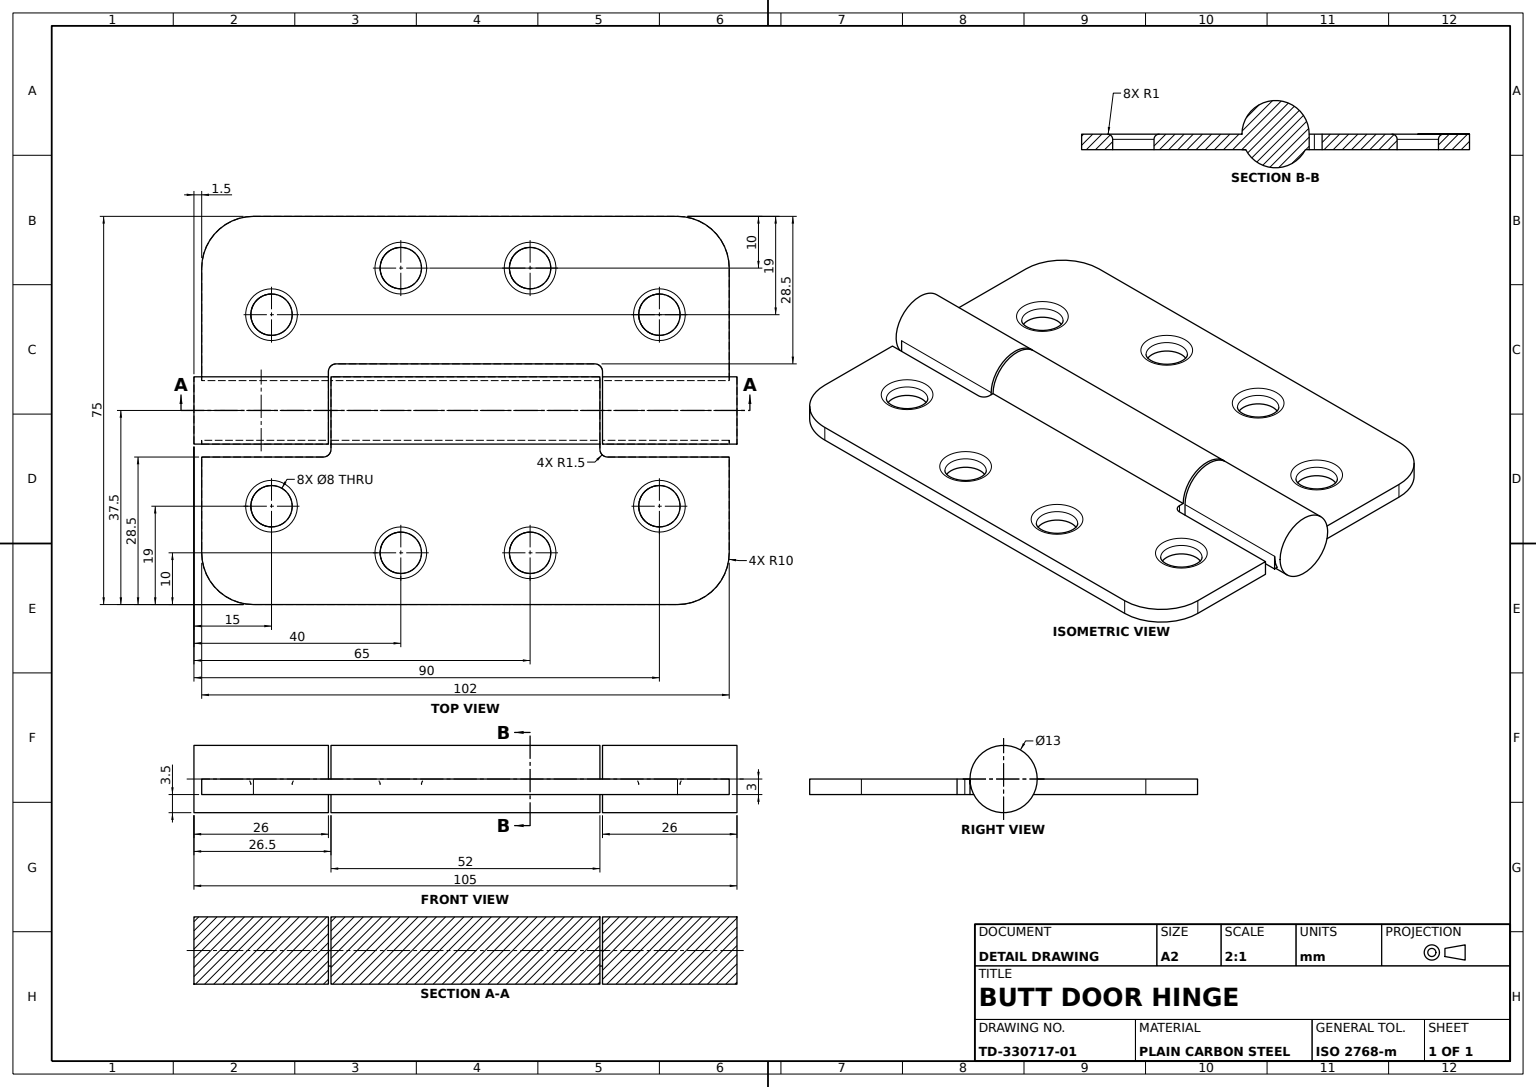
solid
v1 (77.5,-3,-5.766281)
v2 (77.5,-3,5.766281)
e1 v1 v2 CIRCLE(AX(P(77.5,0,0),D(-1,0,0),D(0,0,1)),6.5)
v3 (102,-3,-5.766281)
e2 v1 v3 LINE
v4 (102,0,-6.5)
e3 v4 v3 CIRCLE(AX(P(102,0,0),D(-1,0,0),D(0,0,-1)),6.5)
v5 (103.5,0,-6.5)
e4 v5 v4 LINE
v6 (103.5,0,6.5)
e5 v5 v6 CIRCLE(AX(P(103.5,0,0),D(-1,0,0),D(0,0,1)),6.5)
v7 (102,0,6.5)
e6 v6 v7 LINE
v8 (102,-3,5.766281)
e7 v8 v7 CIRCLE(AX(P(102,0,0),D(-1,0,0),D(0,0,-1)),6.5)
e8 v8 v2 LINE
face CYL(AX(P(77.5,0,0),D(-1,0,0),D(0,0,1)),6.5) [-e1 e2 -e3 -e4 e5 e6 -e7 e8]
v9 (77.5,-3,6.5)
v10 (102,-3,6.5)
e9 v9 v10 LINE
e10 v2 v9 LINE
e11 v10 v8 LINE
face PLANE(AX(P(26,-3,-7.5),D(0,1,0),D(0,0,1))) rev [-e9 -e10 -e8 -e11]
v11 (88.5,-1,-14.5)
v12 (88.5,-1,-22.5)
e12 v11 v12 CIRCLE(AX(P(88.5,-1,-18.5),D(0,1,0),D(0,0,1)),4)
v13 (88.5,-3,-22.5)
e13 v13 v12 LINE
v14 (88.5,-3,-14.5)
e14 v14 v13 CIRCLE(AX(P(88.5,-3,-18.5),D(0,1,0),D(0,0,1)),4)
e15 v14 v11 LINE
face CYL(AX(P(88.5,-3,-18.5),D(0,1,0),D(0,0,1)),4) rev [e12 -e13 -e14 e15]
v15 (13.5,-1,-14.5)
v16 (13.5,-1,-22.5)
e16 v15 v16 CIRCLE(AX(P(13.5,-1,-18.5),D(0,1,0),D(0,0,1)),4)
v17 (13.5,-3,-22.5)
e17 v17 v16 LINE
v18 (13.5,-3,-14.5)
e18 v18 v17 CIRCLE(AX(P(13.5,-3,-18.5),D(0,1,0),D(0,0,1)),4)
e19 v18 v15 LINE
face CYL(AX(P(13.5,-3,-18.5),D(0,1,0),D(0,0,1)),4) rev [e16 -e17 -e18 e19]
v19 (0,-3,5.766281)
v20 (24.5,-3,5.766281)
e20 v19 v20 LINE
v21 (0,0,6.5)
e21 v19 v21 CIRCLE(AX(P(0,0,0),D(-1,0,0),D(0,0,1)),6.5)
v22 (24.5,0,6.5)
e22 v21 v22 LINE
v23 (24.5,6.5,0)
e23 v23 v22 CIRCLE(AX(P(24.5,0,0),D(1,0,0),D(0,1,0)),6.5)
v24 (-1.5,6.5,0)
e24 v24 v23 LINE
v25 (-1.5,-6.5,0)
e25 v24 v25 CIRCLE(AX(P(-1.5,0,0),D(1,0,0),D(0,1,0)),6.5)
v26 (24.5,-6.5,0)
e26 v25 v26 LINE
e27 v20 v26 CIRCLE(AX(P(24.5,0,0),D(1,0,0),D(0,1,0)),6.5)
face CYL(AX(P(24.5,0,0),D(1,0,0),D(0,1,0)),6.5) [-e20 e21 e22 -e23 -e24 e25 e26 -e27]
v27 (26,-3,-9)
v28 (26,0,-9)
e28 v27 v28 LINE
v29 (24.5,0,-7.5)
e29 v29 v28 CIRCLE(AX(P(26,0,-7.5),D(0,-1,0),D(0,0,1)),1.5)
v30 (24.5,-3,-7.5)
e30 v30 v29 LINE
e31 v30 v27 CIRCLE(AX(P(26,-3,-7.5),D(0,-1,0),D(0,0,1)),1.5)
face CYL(AX(P(26,-3,-7.5),D(0,1,0),D(0,0,1)),1.5) rev [e28 -e29 -e30 e31]
v31 (63.5,-3,-31.5)
v32 (63.5,-1,-31.5)
e32 v31 v32 LINE
v33 (63.5,-3,-23.5)
e33 v33 v31 CIRCLE(AX(P(63.5,-3,-27.5),D(0,1,0),D(0,0,1)),4)
v34 (63.5,-1,-23.5)
e34 v33 v34 LINE
e35 v34 v32 CIRCLE(AX(P(63.5,-1,-27.5),D(0,1,0),D(0,0,1)),4)
face CYL(AX(P(63.5,-3,-27.5),D(0,1,0),D(0,0,1)),4) rev [-e32 -e33 e34 e35]
v35 (24.5,-3,-5.766281)
e36 v26 v35 CIRCLE(AX(P(24.5,0,0),D(1,0,0),D(0,1,0)),6.5)
e37 v35 v30 LINE
v36 (24.5,0,-6.5)
e38 v36 v29 LINE
e39 v36 v23 CIRCLE(AX(P(24.5,0,0),D(1,0,0),D(0,1,0)),6.5)
v37 (24.5,-3,6.5)
e40 v37 v22 LINE
e41 v37 v20 LINE
face PLANE(AX(P(24.5,-3,6.5),D(1,0,0),D(0,0,-1))) [e36 e37 e30 -e38 e39 e23 -e40 e41 e27]
v38 (0,-3,6.5)
e42 v38 v37 LINE
e43 v38 v21 LINE
face PLANE(AX(P(0,-3,6.5),D(0,0,1),D(1,0,0))) [e42 e40 -e22 -e43]
e44 v12 v11 CIRCLE(AX(P(88.5,-1,-18.5),D(0,1,0),D(0,0,1)),4)
v39 (88.5,0,-23.5)
e45 v39 v12 CIRCLE(AX(P(88.5,-1,-23.5),D(1,0,0),D(0,0,-1)),1)
v40 (88.5,0,-13.5)
e46 v40 v39 CIRCLE(AX(P(88.5,0,-18.5),D(0,-1,0),D(0,0,1)),5)
e47 v40 v11 CIRCLE(AX(P(88.5,-1,-13.5),D(-1,0,0),D(0,0,1)),1)
face TORUS(AX(P(88.5,-1,-18.5),D(0,1,0),D(0,0,1)),5,1) [-e44 -e45 -e46 e47]
v41 (38.5,-3,-23.5)
v42 (38.5,-3,-31.5)
e48 v41 v42 CIRCLE(AX(P(38.5,-3,-27.5),D(0,1,0),D(0,0,1)),4)
v43 (38.5,-1,-23.5)
e49 v41 v43 LINE
v44 (38.5,-1,-31.5)
e50 v43 v44 CIRCLE(AX(P(38.5,-1,-27.5),D(0,1,0),D(0,0,1)),4)
e51 v42 v44 LINE
face CYL(AX(P(38.5,-3,-27.5),D(0,1,0),D(0,0,1)),4) rev [-e48 e49 e50 -e51]
e52 v44 v43 CIRCLE(AX(P(38.5,-1,-27.5),D(0,1,0),D(0,0,1)),4)
e53 v42 v41 CIRCLE(AX(P(38.5,-3,-27.5),D(0,1,0),D(0,0,1)),4)
face CYL(AX(P(38.5,-3,-27.5),D(0,1,0),D(0,0,1)),4) rev [e51 e52 -e49 -e53]
v45 (0,0,-6.5)
e54 v36 v45 LINE
v46 (0,-3,-5.766281)
e55 v45 v46 CIRCLE(AX(P(0,0,0),D(-1,0,0),D(0,0,1)),6.5)
e56 v35 v46 LINE
e57 v25 v24 CIRCLE(AX(P(-1.5,0,0),D(1,0,0),D(0,1,0)),6.5)
face CYL(AX(P(24.5,0,0),D(1,0,0),D(0,1,0)),6.5) [-e39 e54 e55 -e56 -e36 -e26 e57 e24]
e58 v13 v14 CIRCLE(AX(P(88.5,-3,-18.5),D(0,1,0),D(0,0,1)),4)
face CYL(AX(P(88.5,-3,-18.5),D(0,1,0),D(0,0,1)),4) rev [-e15 -e58 e13 e44]
v47 (63.5,0,-22.5)
v48 (63.5,0,-32.5)
e59 v47 v48 CIRCLE(AX(P(63.5,0,-27.5),D(0,-1,0),D(0,0,1)),5)
e60 v47 v34 CIRCLE(AX(P(63.5,-1,-22.5),D(-1,0,0),D(0,0,1)),1)
e61 v32 v34 CIRCLE(AX(P(63.5,-1,-27.5),D(0,1,0),D(0,0,1)),4)
e62 v48 v32 CIRCLE(AX(P(63.5,-1,-32.5),D(1,0,0),D(0,0,-1)),1)
face TORUS(AX(P(63.5,-1,-27.5),D(0,1,0),D(0,0,1)),5,1) [-e59 e60 -e61 -e62]
v49 (76,0,-9)
e63 v28 v49 LINE
v50 (76,-3,-9)
e64 v27 v50 LINE
e65 v50 v49 LINE
face PLANE(AX(P(26,-3,-9),D(0,0,1),D(1,0,0))) [-e63 -e28 e64 e65]
v51 (10,-3,-37.5)
v52 (10,0,-37.5)
e66 v51 v52 LINE
v53 (92,0,-37.5)
e67 v53 v52 LINE
v54 (92,-3,-37.5)
e68 v54 v53 LINE
e69 v54 v51 LINE
face PLANE(AX(P(92,-3,-37.5),D(0,0,-1),D(-1,0,0))) [e66 -e67 -e68 e69]
v55 (0,0,-27.5)
e70 v55 v45 LINE
v56 (0,-3,-27.5)
e71 v56 v55 LINE
e72 v56 v46 LINE
face PLANE(AX(P(0,-3,0),D(-1,0,0),D(0,0,1))) [-e70 -e71 e72 -e55]
e73 v19 v38 LINE
face PLANE(AX(P(0,-3,0),D(-1,0,0),D(0,0,1))) [e73 e43 -e21]
face PLANE(AX(P(-1.5,0,0),D(-1,0,0),D(0,-1,0))) [-e57 -e25]
e74 v48 v47 CIRCLE(AX(P(63.5,0,-27.5),D(0,-1,0),D(0,0,1)),5)
face TORUS(AX(P(63.5,-1,-27.5),D(0,1,0),D(0,0,1)),5,1) [-e35 -e60 -e74 e62]
e75 v10 v7 LINE
v57 (77.5,0,6.5)
e76 v57 v7 LINE
e77 v9 v57 LINE
face PLANE(AX(P(77.5,-3,6.5),D(0,0,1),D(1,0,0))) [e75 -e76 -e77 e9]
e78 v52 v55 CIRCLE(AX(P(10,0,-27.5),D(0,1,0),D(0,0,1)),10)
e79 v51 v56 CIRCLE(AX(P(10,-3,-27.5),D(0,1,0),D(0,0,1)),10)
face CYL(AX(P(10,-3,-27.5),D(0,1,0),D(0,0,1)),10) [e71 -e78 -e66 e79]
face PLANE(AX(P(26,-3,-7.5),D(0,1,0),D(0,0,1))) rev [e20 -e41 -e42 -e73]
v58 (77.5,-3,-7.5)
e80 v50 v58 CIRCLE(AX(P(76,-3,-7.5),D(0,-1,0),D(0,0,1)),1.5)
v59 (77.5,0,-7.5)
e81 v58 v59 LINE
e82 v49 v59 CIRCLE(AX(P(76,0,-7.5),D(0,-1,0),D(0,0,1)),1.5)
face CYL(AX(P(76,-3,-7.5),D(0,1,0),D(0,0,1)),1.5) rev [e80 e81 -e82 -e65]
v60 (77.5,0,-6.5)
e83 v57 v60 CIRCLE(AX(P(77.5,0,0),D(-1,0,0),D(0,0,1)),6.5)
e84 v6 v5 CIRCLE(AX(P(103.5,0,0),D(-1,0,0),D(0,0,1)),6.5)
e85 v60 v4 LINE
face CYL(AX(P(77.5,0,0),D(-1,0,0),D(0,0,1)),6.5) [-e83 e76 -e6 e84 e4 -e85]
e86 v17 v18 CIRCLE(AX(P(13.5,-3,-18.5),D(0,1,0),D(0,0,1)),4)
e87 v16 v15 CIRCLE(AX(P(13.5,-1,-18.5),D(0,1,0),D(0,0,1)),4)
face CYL(AX(P(13.5,-3,-18.5),D(0,1,0),D(0,0,1)),4) rev [-e19 -e86 e17 e87]
e88 v39 v40 CIRCLE(AX(P(88.5,0,-18.5),D(0,-1,0),D(0,0,1)),5)
v61 (13.5,0,-13.5)
v62 (13.5,0,-23.5)
e89 v61 v62 CIRCLE(AX(P(13.5,0,-18.5),D(0,-1,0),D(0,0,1)),5)
e90 v62 v61 CIRCLE(AX(P(13.5,0,-18.5),D(0,-1,0),D(0,0,1)),5)
e91 v59 v60 LINE
v63 (102,0,-27.5)
e92 v4 v63 LINE
e93 v63 v53 CIRCLE(AX(P(92,0,-27.5),D(0,1,0),D(0,0,1)),10)
v64 (38.5,0,-22.5)
v65 (38.5,0,-32.5)
e94 v64 v65 CIRCLE(AX(P(38.5,0,-27.5),D(0,-1,0),D(0,0,1)),5)
e95 v65 v64 CIRCLE(AX(P(38.5,0,-27.5),D(0,-1,0),D(0,0,1)),5)
face PLANE(AX(P(26,0,-7.5),D(0,1,0),D(0,0,1))) [e88 e46] [e59 e74] [e89 e90] [e63 e82 e91 e85 e92 e93 e67 e78 e70 -e54 e38 e29] [e94 e95]
e96 v62 v16 CIRCLE(AX(P(13.5,-1,-23.5),D(1,0,0),D(0,0,-1)),1)
e97 v61 v15 CIRCLE(AX(P(13.5,-1,-13.5),D(-1,0,0),D(0,0,1)),1)
face TORUS(AX(P(13.5,-1,-18.5),D(0,1,0),D(0,0,1)),5,1) [-e87 -e96 -e89 e97]
e98 v58 v1 LINE
face PLANE(AX(P(77.5,-3,-7.5),D(-1,0,0),D(0,0,1))) [e10 e77 e83 -e91 -e81 e98 e1]
e99 v31 v33 CIRCLE(AX(P(63.5,-3,-27.5),D(0,1,0),D(0,0,1)),4)
face CYL(AX(P(63.5,-3,-27.5),D(0,1,0),D(0,0,1)),4) rev [-e99 e32 e61 -e34]
e100 v64 v43 CIRCLE(AX(P(38.5,-1,-22.5),D(-1,0,0),D(0,0,1)),1)
e101 v65 v44 CIRCLE(AX(P(38.5,-1,-32.5),D(1,0,0),D(0,0,-1)),1)
face TORUS(AX(P(38.5,-1,-27.5),D(0,1,0),D(0,0,1)),5,1) [-e50 -e100 -e95 e101]
face TORUS(AX(P(13.5,-1,-18.5),D(0,1,0),D(0,0,1)),5,1) [-e16 -e97 -e90 e96]
v66 (102,-3,-27.5)
e102 v66 v63 LINE
e103 v66 v54 CIRCLE(AX(P(92,-3,-27.5),D(0,1,0),D(0,0,1)),10)
face CYL(AX(P(92,-3,-27.5),D(0,1,0),D(0,0,1)),10) [-e93 -e102 e103 e68]
e104 v3 v66 LINE
face PLANE(AX(P(26,-3,-7.5),D(0,1,0),D(0,0,1))) rev [e18 e86] [e99 e33] [e58 e14] [-e72 -e79 -e69 -e103 -e104 -e2 -e98 -e80 -e64 -e31 -e37 e56] [e48 e53]
face PLANE(AX(P(102,-3,6.5),D(1,0,0),D(0,0,-1))) [e11 e7 -e75]
face PLANE(AX(P(103.5,0,0),D(-1,0,0),D(0,0,1))) rev [-e84 -e5]
face TORUS(AX(P(88.5,-1,-18.5),D(0,1,0),D(0,0,1)),5,1) [e45 -e12 -e47 -e88]
face PLANE(AX(P(102,-3,6.5),D(1,0,0),D(0,0,-1))) [e3 e104 e102 -e92]
face TORUS(AX(P(38.5,-1,-27.5),D(0,1,0),D(0,0,1)),5,1) [-e52 -e101 -e94 e100]
solid
v67 (25,-3,-6.5)
v68 (25,-3,-5.766281)
e105 v67 v68 LINE
v69 (25,-3,5.766281)
e106 v68 v69 CIRCLE(AX(P(25,0,0),D(-1,0,0),D(0,0,1)),6.5)
v70 (25,-3,7.5)
e107 v69 v70 LINE
v71 (25,0,7.5)
e108 v70 v71 LINE
v72 (25,0,6.5)
e109 v72 v71 LINE
v73 (25,0,-6.5)
e110 v72 v73 CIRCLE(AX(P(25,0,0),D(-1,0,0),D(0,0,1)),6.5)
e111 v67 v73 LINE
face PLANE(AX(P(25,-3,7.5),D(-1,0,0),D(0,0,1))) [e105 e106 e107 e108 -e109 e110 -e111]
v74 (102,0,9)
v75 (78.5,0,9)
e112 v74 v75 LINE
v76 (102,-3,9)
e113 v76 v74 LINE
v77 (78.5,-3,9)
e114 v76 v77 LINE
e115 v77 v75 LINE
face PLANE(AX(P(102,-3,9),D(0,0,-1),D(-1,0,0))) [-e112 -e113 e114 e115]
v78 (88.5,-3,14.5)
v79 (88.5,-1,14.5)
e116 v78 v79 LINE
v80 (88.5,-3,22.5)
e117 v80 v78 CIRCLE(AX(P(88.5,-3,18.5),D(0,1,0),D(0,0,1)),4)
v81 (88.5,-1,22.5)
e118 v80 v81 LINE
e119 v81 v79 CIRCLE(AX(P(88.5,-1,18.5),D(0,1,0),D(0,0,-1)),4)
face CYL(AX(P(88.5,-3,18.5),D(0,1,0),D(0,0,1)),4) rev [-e116 -e117 e118 e119]
v82 (88.5,0,13.5)
v83 (88.5,0,23.5)
e120 v82 v83 CIRCLE(AX(P(88.5,0,18.5),D(0,-1,0),D(0,0,-1)),5)
e121 v79 v82 CIRCLE(AX(P(88.5,-1,13.5),D(-1,0,0),D(0,0,1)),1)
e122 v81 v83 CIRCLE(AX(P(88.5,-1,23.5),D(1,0,0),D(0,0,-1)),1)
face TORUS(AX(P(88.5,-1,18.5),D(0,-1,0),D(0,0,-1)),5,1) [-e120 -e121 -e119 e122]
v84 (77,0,-6.5)
e123 v84 v73 LINE
v85 (77,0,6.5)
e124 v72 v85 LINE
e125 v85 v84 CIRCLE(AX(P(77,0,0),D(-1,0,0),D(0,0,1)),6.5)
face CYL(AX(P(25,0,0),D(-1,0,0),D(0,0,1)),6.5) [e123 -e110 e124 e125]
v86 (13.5,-1,14.5)
v87 (13.5,-1,22.5)
e126 v86 v87 CIRCLE(AX(P(13.5,-1,18.5),D(0,1,0),D(0,0,-1)),4)
v88 (13.5,0,13.5)
e127 v86 v88 CIRCLE(AX(P(13.5,-1,13.5),D(-1,0,0),D(0,0,1)),1)
v89 (13.5,0,23.5)
e128 v89 v88 CIRCLE(AX(P(13.5,0,18.5),D(0,-1,0),D(0,0,-1)),5)
e129 v87 v89 CIRCLE(AX(P(13.5,-1,23.5),D(1,0,0),D(0,0,-1)),1)
face TORUS(AX(P(13.5,-1,18.5),D(0,-1,0),D(0,0,-1)),5,1) [-e126 e127 -e128 -e129]
v90 (38.5,-1,23.5)
v91 (38.5,-1,31.5)
e130 v90 v91 CIRCLE(AX(P(38.5,-1,27.5),D(0,1,0),D(0,0,-1)),4)
v92 (38.5,-3,31.5)
e131 v92 v91 LINE
v93 (38.5,-3,23.5)
e132 v93 v92 CIRCLE(AX(P(38.5,-3,27.5),D(0,1,0),D(0,0,1)),4)
e133 v93 v90 LINE
face CYL(AX(P(38.5,-3,27.5),D(0,1,0),D(0,0,1)),4) rev [e130 -e131 -e132 e133]
e134 v83 v82 CIRCLE(AX(P(88.5,0,18.5),D(0,-1,0),D(0,0,-1)),5)
e135 v79 v81 CIRCLE(AX(P(88.5,-1,18.5),D(0,1,0),D(0,0,-1)),4)
face TORUS(AX(P(88.5,-1,18.5),D(0,-1,0),D(0,0,-1)),5,1) [-e134 -e122 -e135 e121]
v94 (77,-3,7.5)
v95 (77,0,7.5)
e136 v94 v95 LINE
e137 v75 v95 CIRCLE(AX(P(78.5,0,7.5),D(0,-1,0),D(0,0,-1)),1.5)
e138 v77 v94 CIRCLE(AX(P(78.5,-3,7.5),D(0,-1,0),D(0,0,-1)),1.5)
face CYL(AX(P(78.5,-3,7.5),D(0,1,0),D(0,0,1)),1.5) rev [e136 -e137 -e115 e138]
v96 (102,-3,27.5)
e139 v96 v76 LINE
v97 (102,0,27.5)
e140 v97 v74 LINE
e141 v96 v97 LINE
face PLANE(AX(P(102,-3,27.5),D(1,0,0),D(0,0,-1))) [e139 e113 -e140 -e141]
v98 (77,-3,-6.5)
e142 v98 v84 LINE
e143 v95 v85 LINE
v99 (77,-3,5.766281)
e144 v94 v99 LINE
v100 (77,-3,-5.766281)
e145 v100 v99 CIRCLE(AX(P(77,0,0),D(-1,0,0),D(0,0,1)),6.5)
e146 v100 v98 LINE
face PLANE(AX(P(77,-3,-6.5),D(1,0,0),D(0,0,-1))) [e142 -e125 -e143 -e136 e144 -e145 e146]
e147 v100 v68 LINE
e148 v69 v99 LINE
face CYL(AX(P(25,0,0),D(-1,0,0),D(0,0,1)),6.5) [-e147 e145 -e148 -e106]
v101 (63.5,-3,31.5)
v102 (63.5,-3,23.5)
e149 v101 v102 CIRCLE(AX(P(63.5,-3,27.5),D(0,1,0),D(0,0,1)),4)
v103 (63.5,-1,31.5)
e150 v101 v103 LINE
v104 (63.5,-1,23.5)
e151 v103 v104 CIRCLE(AX(P(63.5,-1,27.5),D(0,1,0),D(0,0,-1)),4)
e152 v102 v104 LINE
face CYL(AX(P(63.5,-3,27.5),D(0,1,0),D(0,0,1)),4) rev [-e149 e150 e151 -e152]
v105 (38.5,0,32.5)
e153 v91 v105 CIRCLE(AX(P(38.5,-1,32.5),D(1,0,0),D(0,0,-1)),1)
v106 (38.5,0,22.5)
e154 v90 v106 CIRCLE(AX(P(38.5,-1,22.5),D(-1,0,0),D(0,0,1)),1)
e155 v105 v106 CIRCLE(AX(P(38.5,0,27.5),D(0,-1,0),D(0,0,-1)),5)
face TORUS(AX(P(38.5,-1,27.5),D(0,-1,0),D(0,0,-1)),5,1) [-e153 -e130 e154 -e155]
e156 v87 v86 CIRCLE(AX(P(13.5,-1,18.5),D(0,1,0),D(0,0,-1)),4)
e157 v88 v89 CIRCLE(AX(P(13.5,0,18.5),D(0,-1,0),D(0,0,-1)),5)
face TORUS(AX(P(13.5,-1,18.5),D(0,-1,0),D(0,0,-1)),5,1) [-e127 -e156 e129 -e157]
e158 v92 v93 CIRCLE(AX(P(38.5,-3,27.5),D(0,1,0),D(0,0,1)),4)
e159 v102 v101 CIRCLE(AX(P(63.5,-3,27.5),D(0,1,0),D(0,0,1)),4)
v107 (92,-3,37.5)
e160 v107 v96 CIRCLE(AX(P(92,-3,27.5),D(0,1,0),D(0,0,1)),10)
v108 (10,-3,37.5)
e161 v108 v107 LINE
v109 (0,-3,27.5)
e162 v109 v108 CIRCLE(AX(P(10,-3,27.5),D(0,1,0),D(0,0,-1)),10)
v110 (0,-3,9)
e163 v110 v109 LINE
v111 (23.5,-3,9)
e164 v111 v110 LINE
e165 v70 v111 CIRCLE(AX(P(23.5,-3,7.5),D(0,-1,0),D(0,0,1)),1.5)
e166 v78 v80 CIRCLE(AX(P(88.5,-3,18.5),D(0,1,0),D(0,0,1)),4)
v112 (13.5,-3,14.5)
v113 (13.5,-3,22.5)
e167 v112 v113 CIRCLE(AX(P(13.5,-3,18.5),D(0,1,0),D(0,0,1)),4)
e168 v113 v112 CIRCLE(AX(P(13.5,-3,18.5),D(0,1,0),D(0,0,1)),4)
face PLANE(AX(P(10,-3,27.5),D(0,-1,0),D(0,0,-1))) [e132 e158] [e149 e159] [-e107 e148 -e144 -e138 -e114 -e139 -e160 -e161 -e162 -e163 -e164 -e165] [e166 e117] [e167 e168]
v114 (63.5,0,22.5)
e169 v104 v114 CIRCLE(AX(P(63.5,-1,22.5),D(-1,0,0),D(0,0,1)),1)
v115 (63.5,0,32.5)
e170 v115 v114 CIRCLE(AX(P(63.5,0,27.5),D(0,-1,0),D(0,0,-1)),5)
e171 v103 v115 CIRCLE(AX(P(63.5,-1,32.5),D(1,0,0),D(0,0,-1)),1)
e172 v104 v103 CIRCLE(AX(P(63.5,-1,27.5),D(0,1,0),D(0,0,-1)),4)
face TORUS(AX(P(63.5,-1,27.5),D(0,-1,0),D(0,0,-1)),5,1) [e169 -e170 -e171 -e172]
face CYL(AX(P(63.5,-3,27.5),D(0,1,0),D(0,0,1)),4) rev [-e159 e152 e172 -e150]
v116 (23.5,0,9)
e173 v111 v116 LINE
e174 v71 v116 CIRCLE(AX(P(23.5,0,7.5),D(0,-1,0),D(0,0,1)),1.5)
face CYL(AX(P(23.5,-3,7.5),D(0,1,0),D(0,0,1)),1.5) rev [e165 e173 -e174 -e108]
v117 (92,0,37.5)
e175 v117 v97 CIRCLE(AX(P(92,0,27.5),D(0,1,0),D(0,0,1)),10)
e176 v107 v117 LINE
face CYL(AX(P(92,-3,27.5),D(0,1,0),D(0,0,1)),10) [e160 e141 -e175 -e176]
v118 (10,0,37.5)
e177 v108 v118 LINE
v119 (0,0,27.5)
e178 v119 v118 CIRCLE(AX(P(10,0,27.5),D(0,1,0),D(0,0,-1)),10)
e179 v109 v119 LINE
face CYL(AX(P(10,-3,27.5),D(0,1,0),D(0,0,1)),10) [e162 e177 -e178 -e179]
v120 (0,0,9)
e180 v116 v120 LINE
e181 v120 v119 LINE
e182 v118 v117 LINE
e183 v106 v105 CIRCLE(AX(P(38.5,0,27.5),D(0,-1,0),D(0,0,-1)),5)
e184 v114 v115 CIRCLE(AX(P(63.5,0,27.5),D(0,-1,0),D(0,0,-1)),5)
face PLANE(AX(P(10,0,27.5),D(0,-1,0),D(0,0,-1))) rev [e134 e120] [e109 e174 e180 e181 e178 e182 e175 e140 e112 e137 e143 -e124] [e155 e183] [e157 e128] [e184 e170]
e185 v110 v120 LINE
face PLANE(AX(P(0,-3,9),D(0,0,-1),D(-1,0,0))) [-e180 -e173 e164 e185]
e186 v113 v87 LINE
e187 v112 v86 LINE
face CYL(AX(P(13.5,-3,18.5),D(0,1,0),D(0,0,1)),4) rev [e186 e156 -e187 -e168]
face CYL(AX(P(88.5,-3,18.5),D(0,1,0),D(0,0,1)),4) rev [-e118 -e166 e116 e135]
face PLANE(AX(P(10,-3,37.5),D(0,0,1),D(1,0,0))) [-e182 -e177 e161 e176]
e188 v98 v67 LINE
face PLANE(AX(P(10,-3,27.5),D(0,-1,0),D(0,0,-1))) [-e146 e147 -e105 -e188]
face PLANE(AX(P(0,-3,9),D(-1,0,0),D(0,0,1))) [-e185 e163 e179 -e181]
face TORUS(AX(P(63.5,-1,27.5),D(0,-1,0),D(0,0,-1)),5,1) [-e169 -e151 e171 -e184]
face CYL(AX(P(13.5,-3,18.5),D(0,1,0),D(0,0,1)),4) rev [e187 e126 -e186 -e167]
e189 v91 v90 CIRCLE(AX(P(38.5,-1,27.5),D(0,1,0),D(0,0,-1)),4)
face TORUS(AX(P(38.5,-1,27.5),D(0,-1,0),D(0,0,-1)),5,1) [-e154 -e189 e153 -e183]
face PLANE(AX(P(25,-3,-6.5),D(0,0,-1),D(-1,0,0))) [e111 -e123 -e142 e188]
face CYL(AX(P(38.5,-3,27.5),D(0,1,0),D(0,0,1)),4) rev [e131 e189 -e133 -e158]
